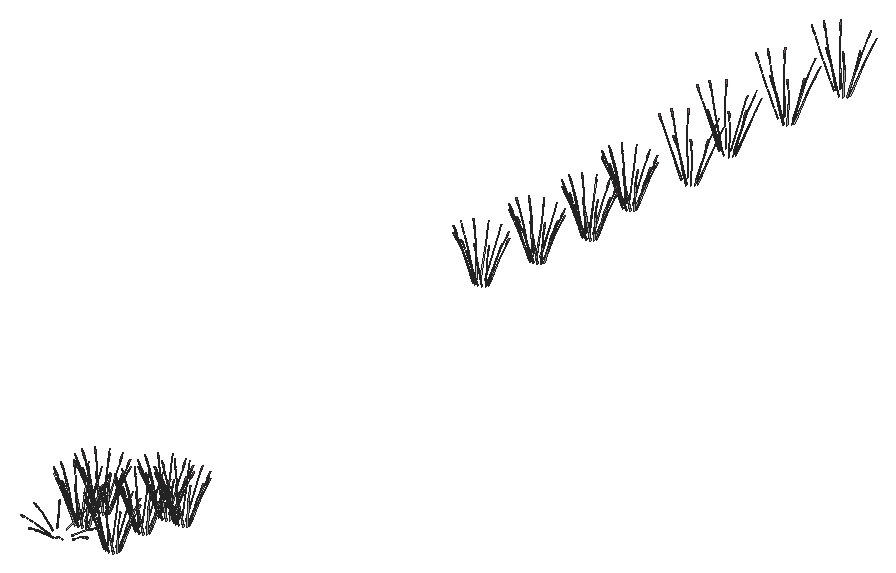
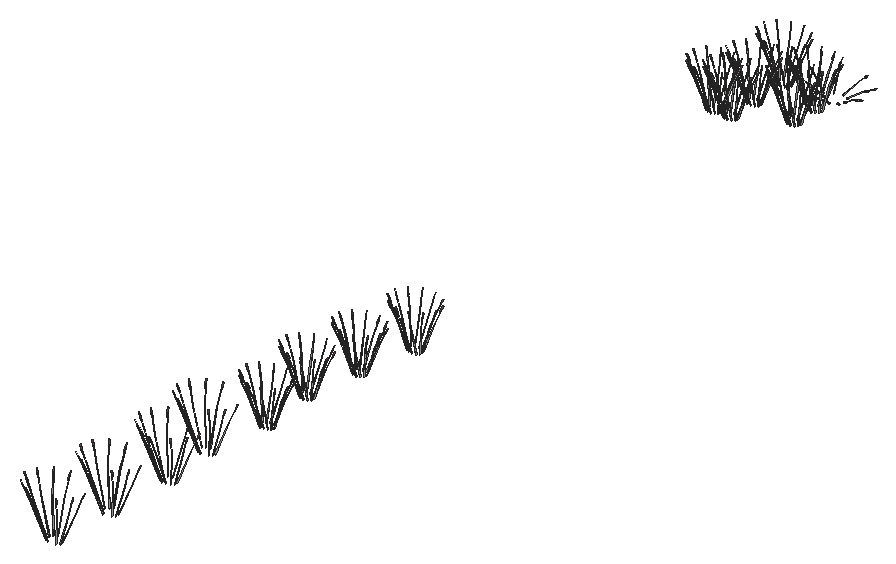
# SketchUp Ruby script. Lengths in inches.
U = 1.inch
M = Sketchup.active_model
def pt(a) = Geom::Point3d.new(a.map { |v| v * U })
def face(e, loops, mat)
  f = e.add_face(loops[0].map { |a| pt(a) })
  loops[1..].each { |l| e.add_face(l.map { |a| pt(a) }).erase! }
  f.material = f.back_material = mat if mat
  f
end
# faces: each face lists its corners as indices into pts; further lists are holes
def faces(e, pts, list, mat = nil) = list.each { |f| face(e, (f[0].is_a?(Array) ? f : [f]).map { |l| l.map { |i| pts[i] } }, mat) }
# xy, xz, yz: faces in a plane at the given z, y or x. An outline is a flat list of corners, or four numbers for a rectangle; further outlines are holes
def ring(l) = l.size == 4 ? [[l[0], l[1]], [l[2], l[1]], [l[2], l[3]], [l[0], l[3]]] : l.each_slice(2).to_a
def flat(e, list, mat, &to3) = list.each { |f| face(e, (f[0].is_a?(Array) ? f : [f]).map { |l| ring(l).map { |u, v| to3.(u, v) } }, mat) }
def xy(e, z, list, mat = nil) = flat(e, list, mat) { |x, y| [x, y, z] }
def xz(e, y, list, mat = nil) = flat(e, list, mat) { |x, z| [x, y, z] }
def yz(e, x, list, mat = nil) = flat(e, list, mat) { |y, z| [x, y, z] }
def lines(e, pts, list) = list.each { |a, b| e.add_line(pt(pts[a]), pt(pts[b])) }
# prism: a flat outline (further loops are holes) pulled along v
def prism(e, loops, v, mat = nil)
  f = face(e, loops, mat); d = Geom::Vector3d.new(v.map { |x| x * U })
  f.pushpull(f.normal.samedirection?(d) ? d.length : -d.length)
end
def box(e, o, s, mat = nil) = prism(e, [[o, [o[0] + s[0], o[1], o[2]], [o[0] + s[0], o[1] + s[1], o[2]], [o[0], o[1] + s[1], o[2]]]], [0, 0, s[2]], mat)
def at(x, y, z, deg = 0) = Geom::Transformation.translation(pt([x, y, z])) * Geom::Transformation.rotation(ORIGIN, Z_AXIS, deg.degrees)
def axes(o, x, y, z) = Geom::Transformation.new([*x, 0, *y, 0, *z, 0, *pt(o).to_a, 1])
def part(name) = M.definitions.add(name)
# library, detail: a bought-in or finely detailed component or shape, given as its bounding box
def library(name, o, s) = part(name).tap { |d| box(d.entities, o, s) }
def detail(e, o, s) = box(e.add_group.entities, o, s)
def put(e, d, t, mat = nil) = e.add_instance(d, t).tap { |i| i.material = mat if mat }
def group(e, t, mat = nil) = e.add_group.tap { |g| g.transformation = t; g.material = mat if mat }.entities
root = M.entities
M.materials.add("LightPink_Translucent").color = [144, 107, 117]
c1 = part("blade")
p = [[2.15,0.21,22],[0,0.17,0],[0.09,0.45,0],[2.18,0.31,22],[2.29,0.31,22],[0.38,0.45,0],
  [2.48,0.24,33],[2.49,0.24,33],[2.48,0.22,33]]
faces(c1.entities,p,[[0,1,2,3],[4,5,2,3],[6,3,4,7],[8,0,3,6]])
c2 = part("seeds")
p = [[0.3,-0.1,1.38],[-0.01,-0.03,1.59],[-0.01,-0.03,0.03],[0.14,-0.07,-0.07],[0.29,-0.03,3],[0.15,0.01,3.11]]
faces(c2.entities,p,[[0,1,2,3],[1,0,4,5]],"LightPink_Translucent")
c3 = part("blade with seeds")
put(c3.entities,c1,at(0,0,0))
put(c3.entities,c2,axes([2.4,0.25,30.99],[1.5799,-0.05474,1.17369],[-0.12525,1.92788,0.29478],[-0.07173,-0.02425,1.56792]))
put(root,c3,axes([53.96,597.61,46.73],[-0.90362,0.68241,0.48003],[-0.77932,-0.72471,0.3958],[0.42395,0.12588,0.9933]))
put(root,c3,axes([55.23,595.46,46.73],[-0.34623,0.9443,0.48003],[-1.13828,-0.3229,0.3958],[0.44763,-0.05675,0.9933]))
put(root,c3,axes([44.01,596.27,46.73],[-0.30393,-0.95317,0.48003],[1.19224,-0.16542,0.3958],[-0.35138,0.22417,0.9933]))
put(root,c3,axes([45.75,598.19,46.73],[-0.87265,-0.70663,0.48003],[0.92674,-0.60943,0.3958],[-0.16097,0.33153,0.9933]))
put(root,c3,axes([53.22,591.18,46.73],[0.87265,0.70663,0.48003],[-0.92674,0.60943,0.3958],[0.16097,-0.33153,0.9933]))
put(root,c3,axes([43.73,593.91,46.73],[0.34623,-0.9443,0.48003],[1.13828,0.3229,0.3958],[-0.44763,0.05675,0.9933]))
put(root,c3,axes([54.96,593.11,46.73],[0.30393,0.95317,0.48003],[-1.19224,0.16542,0.3958],[0.35138,-0.22417,0.9933]))
put(root,c3,axes([51.5,598.97,46.73],[-1.21888,0.23767,0.48003],[-0.21154,-0.93233,0.3958],[0.28666,0.27478,0.9933]))
put(root,c3,axes([53.27,639.2,46.73],[1.20755,0.27075,0.48003],[-0.41292,0.89013,0.3958],[-0.07257,-0.35005,0.9933]))
put(root,c3,axes([56.76,646.62,46.73],[-0.90362,0.68241,0.48003],[-0.77932,-0.72471,0.3958],[0.42395,0.12588,0.9933]))
put(root,c3,axes([58.02,644.47,46.73],[-0.34623,0.9443,0.48003],[-1.13828,-0.3229,0.3958],[0.44763,-0.05675,0.9933]))
put(root,c3,axes([46.8,645.27,46.73],[-0.30393,-0.95317,0.48003],[1.19224,-0.16542,0.3958],[-0.35138,0.22417,0.9933]))
put(root,c3,axes([48.54,647.2,46.73],[-0.87265,-0.70663,0.48003],[0.92674,-0.60943,0.3958],[-0.16097,0.33153,0.9933]))
put(root,c3,axes([56.01,640.19,46.73],[0.87265,0.70663,0.48003],[-0.92674,0.60943,0.3958],[0.16097,-0.33153,0.9933]))
put(root,c3,axes([46.52,642.92,46.73],[0.34623,-0.9443,0.48003],[1.13828,0.3229,0.3958],[-0.44763,0.05675,0.9933]))
put(root,c3,axes([57.75,642.12,46.73],[0.30393,0.95317,0.48003],[-1.19224,0.16542,0.3958],[0.35138,-0.22417,0.9933]))
put(root,c3,axes([54.29,647.98,46.73],[-1.21888,0.23767,0.48003],[-0.21154,-0.93233,0.3958],[0.28666,0.27478,0.9933]))
put(root,c3,axes([57.81,683.53,46.73],[1.20755,0.27075,0.48003],[-0.41292,0.89013,0.3958],[-0.07257,-0.35005,0.9933]))
put(root,c3,axes([61.3,690.95,46.73],[-0.90362,0.68241,0.48003],[-0.77932,-0.72471,0.3958],[0.42395,0.12588,0.9933]))
put(root,c3,axes([62.5625,688.8,46.73],[-0.34623,0.9443,0.48003],[-1.13828,-0.3229,0.3958],[0.44763,-0.05675,0.9933]))
put(root,c3,axes([51.34,689.6,46.73],[-0.30393,-0.95317,0.48003],[1.19224,-0.16542,0.3958],[-0.35138,0.22417,0.9933]))
put(root,c3,axes([53.08,691.53,46.73],[-0.87265,-0.70663,0.48003],[0.92674,-0.60943,0.3958],[-0.16097,0.33153,0.9933]))
put(root,c3,axes([60.55,684.52,46.73],[0.87265,0.70663,0.48003],[-0.92674,0.60943,0.3958],[0.16097,-0.33153,0.9933]))
put(root,c3,axes([51.06,687.25,46.73],[0.34623,-0.9443,0.48003],[1.13828,0.3229,0.3958],[-0.44763,0.05675,0.9933]))
put(root,c3,axes([62.29,686.45,46.73],[0.30393,0.95317,0.48003],[-1.19224,0.16542,0.3958],[0.35138,-0.22417,0.9933]))
put(root,c3,axes([58.83,692.31,46.73],[-1.21888,0.23767,0.48003],[-0.21154,-0.93233,0.3958],[0.28666,0.27478,0.9933]))
put(root,c3,axes([54.3,551.37,46.73],[1.20755,0.27075,0.48003],[-0.41292,0.89013,0.3958],[-0.07257,-0.35005,0.9933]))
put(root,c3,axes([57.79,558.78,46.73],[-0.90362,0.68241,0.48003],[-0.77932,-0.72471,0.3958],[0.42395,0.12588,0.9933]))
put(root,c3,axes([59.0625,556.64,46.73],[-0.34623,0.9443,0.48003],[-1.13828,-0.3229,0.3958],[0.44763,-0.05675,0.9933]))
put(root,c3,axes([47.84,557.44,46.73],[-0.30393,-0.95317,0.48003],[1.19224,-0.16542,0.3958],[-0.35138,0.22417,0.9933]))
put(root,c3,axes([49.58,559.37,46.73],[-0.87265,-0.70663,0.48003],[0.92674,-0.60943,0.3958],[-0.16097,0.33153,0.9933]))
put(root,c3,axes([57.05,552.36,46.73],[0.87265,0.70663,0.48003],[-0.92674,0.60943,0.3958],[0.16097,-0.33153,0.9933]))
put(root,c3,axes([47.5625,555.09,46.73],[0.34623,-0.9443,0.48003],[1.13828,0.3229,0.3958],[-0.44763,0.05675,0.9933]))
put(root,c3,axes([58.79,554.29,46.73],[0.30393,0.95317,0.48003],[-1.19224,0.16542,0.3958],[0.35138,-0.22417,0.9933]))
put(root,c3,axes([55.33,560.14,46.73],[-1.21888,0.23767,0.48003],[-0.21154,-0.93233,0.3958],[0.28666,0.27478,0.9933]))
put(root,c3,axes([23.85,22.0625,46.97],[-0.20012,0.13446,1.74944],[0.01702,0.98243,-0.27667],[-0.45871,0.12776,0.14031]))
put(root,c3,axes([39.17,21.75,46.97],[0.17006,-0.15775,1.74944],[-0.21766,-0.96766,-0.27667],[0.42669,-0.18347,0.14031]))
put(root,c3,axes([35.52,24.54,46.97],[0.26289,-0.01751,1.74944],[0.72108,-0.8046,-0.27667],[0.46761,0.10621,0.14031]))
put(root,c3,axes([35.54,17.54,46.97],[-0.01183,-0.20612,1.74944],[-0.99913,-0.59572,-0.27667],[0.15447,-0.36112,0.14031]))
put(root,c3,axes([23.89,25.73,46.97],[-0.03046,0.20495,1.74944],[0.86449,0.71297,-0.27667],[-0.22632,0.33716,0.14031]))
put(root,c3,axes([28.86,28.27,46.97],[0.15534,0.16677,1.74944],[1.25362,0.06552,-0.27667],[0.12606,0.3678,0.14031]))
put(root,c3,axes([29.92,15.76,46.97],[-0.18744,-0.14521,1.74944],[-1.25089,0.09206,-0.27667],[-0.19964,-0.34731,0.14031]))
put(root,c3,axes([25.82,17.35,46.97],[-0.26368,-0.00731,1.74944],[-0.83946,0.73103,-0.27667],[-0.44791,-0.14937,0.14031]))
put(root,c3,axes([31.05,42.08,47.05],[0.36946,-0.79643,0.35414],[1.07787,0.23229,-0.4572],[0.09883,0.32066,0.87481]))
put(root,c3,axes([33,34.39,47.05],[-0.36946,0.79643,0.35414],[-1.07787,-0.23229,-0.4572],[-0.09883,-0.32066,0.87481]))
put(root,c3,axes([35.79,40.82,47.05],[-0.69728,-0.64842,0.35414],[0.79619,-0.61382,-0.4572],[0.40453,0.09339,0.87481]))
put(root,c3,axes([36.94,39,47.05],[-1.01846,-0.28891,0.35414],[0.29705,-0.84289,-0.4572],[0.41005,-0.07729,0.87481]))
put(root,c3,axes([28.26,35.65,47.05],[0.69728,0.64842,0.35414],[-0.79619,0.61382,-0.4572],[-0.40453,-0.09339,0.87481]))
put(root,c3,axes([28.72,41.18,47.05],[0.82919,-0.54528,0.35414],[0.78493,0.62262,-0.4572],[-0.11943,0.31634,0.87481]))
put(root,c3,axes([27.28,39.49,47.05],[1.06674,-0.14801,0.35414],[0.28168,0.84611,-0.4572],[-0.30569,0.22726,0.87481]))
put(root,c3,axes([33.64,41.94,47.05],[-0.18927,-0.83419,0.35414],[1.08199,-0.22027,-0.4572],[0.29062,0.23905,0.87481]))
put(root,c3,axes([36.77,36.98,47.05],[-1.06674,0.14801,0.35414],[-0.28168,-0.84611,-0.4572],[0.30569,-0.22726,0.87481]))
put(root,c3,axes([27.11,37.47,47.05],[1.01846,0.28891,0.35414],[-0.29705,0.84289,-0.4572],[-0.41005,0.07729,0.87481]))
put(root,c3,axes([35.33,35.29,47.05],[-0.82919,0.54528,0.35414],[-0.78493,-0.62262,-0.4572],[0.11943,-0.31634,0.87481]))
put(root,c3,axes([30.42,34.53,47.05],[0.18927,0.83419,0.35414],[-1.08199,0.22027,-0.4572],[-0.29062,-0.23905,0.87481]))
put(root,c3,axes([30.75,61.11,47.05],[0.36946,-0.79643,0.35414],[1.07787,0.23229,-0.4572],[0.09883,0.32066,0.87481]))
put(root,c3,axes([32.71,53.42,47.05],[-0.36946,0.79643,0.35414],[-1.07787,-0.23229,-0.4572],[-0.09883,-0.32066,0.87481]))
put(root,c3,axes([35.49,59.85,47.05],[-0.69728,-0.64842,0.35414],[0.79619,-0.61382,-0.4572],[0.40453,0.09339,0.87481]))
put(root,c3,axes([36.64,58.03,47.05],[-1.01846,-0.28891,0.35414],[0.29705,-0.84289,-0.4572],[0.41005,-0.07729,0.87481]))
put(root,c3,axes([27.96,54.68,47.05],[0.69728,0.64842,0.35414],[-0.79619,0.61382,-0.4572],[-0.40453,-0.09339,0.87481]))
put(root,c3,axes([28.43,60.21,47.05],[0.82919,-0.54528,0.35414],[0.78493,0.62262,-0.4572],[-0.11943,0.31634,0.87481]))
put(root,c3,axes([26.99,58.52,47.05],[1.06674,-0.14801,0.35414],[0.28168,0.84611,-0.4572],[-0.30569,0.22726,0.87481]))
put(root,c3,axes([33.34,60.97,47.05],[-0.18927,-0.83419,0.35414],[1.08199,-0.22027,-0.4572],[0.29062,0.23905,0.87481]))
put(root,c3,axes([36.47,56.01,47.05],[-1.06674,0.14801,0.35414],[-0.28168,-0.84611,-0.4572],[0.30569,-0.22726,0.87481]))
put(root,c3,axes([26.82,56.5,47.05],[1.01846,0.28891,0.35414],[-0.29705,0.84289,-0.4572],[-0.41005,0.07729,0.87481]))
put(root,c3,axes([35.03,54.32,47.05],[-0.82919,0.54528,0.35414],[-0.78493,-0.62262,-0.4572],[0.11943,-0.31634,0.87481]))
put(root,c3,axes([30.12,53.55,47.05],[0.18927,0.83419,0.35414],[-1.08199,0.22027,-0.4572],[-0.29062,-0.23905,0.87481]))
put(root,c3,axes([62.52,30.08,47.05],[0.36946,-0.79643,0.35414],[1.07787,0.23229,-0.4572],[0.09883,0.32066,0.87481]))
put(root,c3,axes([64.48,22.39,47.05],[-0.36946,0.79643,0.35414],[-1.07787,-0.23229,-0.4572],[-0.09883,-0.32066,0.87481]))
put(root,c3,axes([67.26,28.82,47.05],[-0.69728,-0.64842,0.35414],[0.79619,-0.61382,-0.4572],[0.40453,0.09339,0.87481]))
put(root,c3,axes([68.41,27,47.05],[-1.01846,-0.28891,0.35414],[0.29705,-0.84289,-0.4572],[0.41005,-0.07729,0.87481]))
put(root,c3,axes([59.73,23.65,47.05],[0.69728,0.64842,0.35414],[-0.79619,0.61382,-0.4572],[-0.40453,-0.09339,0.87481]))
put(root,c3,axes([60.2,29.18,47.05],[0.82919,-0.54528,0.35414],[0.78493,0.62262,-0.4572],[-0.11943,0.31634,0.87481]))
put(root,c3,axes([58.76,27.49,47.05],[1.06674,-0.14801,0.35414],[0.28168,0.84611,-0.4572],[-0.30569,0.22726,0.87481]))
put(root,c3,axes([65.11,29.94,47.05],[-0.18927,-0.83419,0.35414],[1.08199,-0.22027,-0.4572],[0.29062,0.23905,0.87481]))
put(root,c3,axes([68.24,24.98,47.05],[-1.06674,0.14801,0.35414],[-0.28168,-0.84611,-0.4572],[0.30569,-0.22726,0.87481]))
put(root,c3,axes([58.59,25.47,47.05],[1.01846,0.28891,0.35414],[-0.29705,0.84289,-0.4572],[-0.41005,0.07729,0.87481]))
put(root,c3,axes([66.8,23.29,47.05],[-0.82919,0.54528,0.35414],[-0.78493,-0.62262,-0.4572],[0.11943,-0.31634,0.87481]))
put(root,c3,axes([61.89,22.53,47.05],[0.18927,0.83419,0.35414],[-1.08199,0.22027,-0.4572],[-0.29062,-0.23905,0.87481]))
put(root,c3,axes([62.3125,57.36,47.05],[0.36946,-0.79643,0.35414],[1.07787,0.23229,-0.4572],[0.09883,0.32066,0.87481]))
put(root,c3,axes([64.27,49.68,47.05],[-0.36946,0.79643,0.35414],[-1.07787,-0.23229,-0.4572],[-0.09883,-0.32066,0.87481]))
put(root,c3,axes([67.06,56.1,47.05],[-0.69728,-0.64842,0.35414],[0.79619,-0.61382,-0.4572],[0.40453,0.09339,0.87481]))
put(root,c3,axes([68.2,54.28,47.05],[-1.01846,-0.28891,0.35414],[0.29705,-0.84289,-0.4572],[0.41005,-0.07729,0.87481]))
put(root,c3,axes([59.53,50.9375,47.05],[0.69728,0.64842,0.35414],[-0.79619,0.61382,-0.4572],[-0.40453,-0.09339,0.87481]))
put(root,c3,axes([59.99,56.47,47.05],[0.82919,-0.54528,0.35414],[0.78493,0.62262,-0.4572],[-0.11943,0.31634,0.87481]))
put(root,c3,axes([58.55,54.78,47.05],[1.06674,-0.14801,0.35414],[0.28168,0.84611,-0.4572],[-0.30569,0.22726,0.87481]))
put(root,c3,axes([64.9,57.23,47.05],[-0.18927,-0.83419,0.35414],[1.08199,-0.22027,-0.4572],[0.29062,0.23905,0.87481]))
put(root,c3,axes([68.03,52.26,47.05],[-1.06674,0.14801,0.35414],[-0.28168,-0.84611,-0.4572],[0.30569,-0.22726,0.87481]))
put(root,c3,axes([58.38,52.76,47.05],[1.01846,0.28891,0.35414],[-0.29705,0.84289,-0.4572],[-0.41005,0.07729,0.87481]))
put(root,c3,axes([66.59,50.58,47.05],[-0.82919,0.54528,0.35414],[-0.78493,-0.62262,-0.4572],[0.11943,-0.31634,0.87481]))
put(root,c3,axes([61.68,49.8125,47.05],[0.18927,0.83419,0.35414],[-1.08199,0.22027,-0.4572],[-0.29062,-0.23905,0.87481]))
put(root,c3,axes([62.3125,78.08,47.05],[0.36946,-0.79643,0.35414],[1.07787,0.23229,-0.4572],[0.09883,0.32066,0.87481]))
put(root,c3,axes([64.27,70.39,47.05],[-0.36946,0.79643,0.35414],[-1.07787,-0.23229,-0.4572],[-0.09883,-0.32066,0.87481]))
put(root,c3,axes([67.06,76.82,47.05],[-0.69728,-0.64842,0.35414],[0.79619,-0.61382,-0.4572],[0.40453,0.09339,0.87481]))
put(root,c3,axes([68.2,75,47.05],[-1.01846,-0.28891,0.35414],[0.29705,-0.84289,-0.4572],[0.41005,-0.07729,0.87481]))
put(root,c3,axes([59.53,71.65,47.05],[0.69728,0.64842,0.35414],[-0.79619,0.61382,-0.4572],[-0.40453,-0.09339,0.87481]))
put(root,c3,axes([59.99,77.18,47.05],[0.82919,-0.54528,0.35414],[0.78493,0.62262,-0.4572],[-0.11943,0.31634,0.87481]))
put(root,c3,axes([58.55,75.49,47.05],[1.06674,-0.14801,0.35414],[0.28168,0.84611,-0.4572],[-0.30569,0.22726,0.87481]))
put(root,c3,axes([64.9,77.94,47.05],[-0.18927,-0.83419,0.35414],[1.08199,-0.22027,-0.4572],[0.29062,0.23905,0.87481]))
put(root,c3,axes([68.03,72.98,47.05],[-1.06674,0.14801,0.35414],[-0.28168,-0.84611,-0.4572],[0.30569,-0.22726,0.87481]))
put(root,c3,axes([58.38,73.47,47.05],[1.01846,0.28891,0.35414],[-0.29705,0.84289,-0.4572],[-0.41005,0.07729,0.87481]))
put(root,c3,axes([66.59,71.29,47.05],[-0.82919,0.54528,0.35414],[-0.78493,-0.62262,-0.4572],[0.11943,-0.31634,0.87481]))
put(root,c3,axes([61.68,70.53,47.05],[0.18927,0.83419,0.35414],[-1.08199,0.22027,-0.4572],[-0.29062,-0.23905,0.87481]))
put(root,c3,axes([74.3125,78.08,47.05],[0.36946,-0.79643,0.35414],[1.07787,0.23229,-0.4572],[0.09883,0.32066,0.87481]))
put(root,c3,axes([76.27,70.39,47.05],[-0.36946,0.79643,0.35414],[-1.07787,-0.23229,-0.4572],[-0.09883,-0.32066,0.87481]))
put(root,c3,axes([79.06,76.82,47.05],[-0.69728,-0.64842,0.35414],[0.79619,-0.61382,-0.4572],[0.40453,0.09339,0.87481]))
put(root,c3,axes([80.2,75,47.05],[-1.01846,-0.28891,0.35414],[0.29705,-0.84289,-0.4572],[0.41005,-0.07729,0.87481]))
put(root,c3,axes([71.53,71.65,47.05],[0.69728,0.64842,0.35414],[-0.79619,0.61382,-0.4572],[-0.40453,-0.09339,0.87481]))
put(root,c3,axes([71.99,77.18,47.05],[0.82919,-0.54528,0.35414],[0.78493,0.62262,-0.4572],[-0.11943,0.31634,0.87481]))
put(root,c3,axes([70.55,75.49,47.05],[1.06674,-0.14801,0.35414],[0.28168,0.84611,-0.4572],[-0.30569,0.22726,0.87481]))
put(root,c3,axes([76.9,77.94,47.05],[-0.18927,-0.83419,0.35414],[1.08199,-0.22027,-0.4572],[0.29062,0.23905,0.87481]))
put(root,c3,axes([80.03,72.98,47.05],[-1.06674,0.14801,0.35414],[-0.28168,-0.84611,-0.4572],[0.30569,-0.22726,0.87481]))
put(root,c3,axes([70.38,73.47,47.05],[1.01846,0.28891,0.35414],[-0.29705,0.84289,-0.4572],[-0.41005,0.07729,0.87481]))
put(root,c3,axes([78.59,71.29,47.05],[-0.82919,0.54528,0.35414],[-0.78493,-0.62262,-0.4572],[0.11943,-0.31634,0.87481]))
put(root,c3,axes([73.68,70.53,47.05],[0.18927,0.83419,0.35414],[-1.08199,0.22027,-0.4572],[-0.29062,-0.23905,0.87481]))
put(root,c3,axes([33.47,396.8125,47.05],[0.36946,-0.79643,0.35414],[1.07787,0.23229,-0.4572],[0.09883,0.32066,0.87481]))
put(root,c3,axes([35.43,389.13,47.05],[-0.36946,0.79643,0.35414],[-1.07787,-0.23229,-0.4572],[-0.09883,-0.32066,0.87481]))
put(root,c3,axes([38.22,395.56,47.05],[-0.69728,-0.64842,0.35414],[0.79619,-0.61382,-0.4572],[0.40453,0.09339,0.87481]))
put(root,c3,axes([39.36,393.74,47.05],[-1.01846,-0.28891,0.35414],[0.29705,-0.84289,-0.4572],[0.41005,-0.07729,0.87481]))
put(root,c3,axes([30.68,390.39,47.05],[0.69728,0.64842,0.35414],[-0.79619,0.61382,-0.4572],[-0.40453,-0.09339,0.87481]))
put(root,c3,axes([31.15,395.92,47.05],[0.82919,-0.54528,0.35414],[0.78493,0.62262,-0.4572],[-0.11943,0.31634,0.87481]))
put(root,c3,axes([29.71,394.23,47.05],[1.06674,-0.14801,0.35414],[0.28168,0.84611,-0.4572],[-0.30569,0.22726,0.87481]))
put(root,c3,axes([36.06,396.68,47.05],[-0.18927,-0.83419,0.35414],[1.08199,-0.22027,-0.4572],[0.29062,0.23905,0.87481]))
put(root,c3,axes([39.19,391.71,47.05],[-1.06674,0.14801,0.35414],[-0.28168,-0.84611,-0.4572],[0.30569,-0.22726,0.87481]))
put(root,c3,axes([29.54,392.21,47.05],[1.01846,0.28891,0.35414],[-0.29705,0.84289,-0.4572],[-0.41005,0.07729,0.87481]))
put(root,c3,axes([37.75,390.03,47.05],[-0.82919,0.54528,0.35414],[-0.78493,-0.62262,-0.4572],[0.11943,-0.31634,0.87481]))
put(root,c3,axes([32.84,389.26,47.05],[0.18927,0.83419,0.35414],[-1.08199,0.22027,-0.4572],[-0.29062,-0.23905,0.87481]))
put(root,c3,axes([41.625,436.51,47.05],[0.36946,-0.79643,0.35414],[1.07787,0.23229,-0.4572],[0.09883,0.32066,0.87481]))
put(root,c3,axes([43.58,428.82,47.05],[-0.36946,0.79643,0.35414],[-1.07787,-0.23229,-0.4572],[-0.09883,-0.32066,0.87481]))
put(root,c3,axes([46.37,435.25,47.05],[-0.69728,-0.64842,0.35414],[0.79619,-0.61382,-0.4572],[0.40453,0.09339,0.87481]))
put(root,c3,axes([47.52,433.43,47.05],[-1.01846,-0.28891,0.35414],[0.29705,-0.84289,-0.4572],[0.41005,-0.07729,0.87481]))
put(root,c3,axes([38.84,430.08,47.05],[0.69728,0.64842,0.35414],[-0.79619,0.61382,-0.4572],[-0.40453,-0.09339,0.87481]))
put(root,c3,axes([39.3,435.61,47.05],[0.82919,-0.54528,0.35414],[0.78493,0.62262,-0.4572],[-0.11943,0.31634,0.87481]))
put(root,c3,axes([37.86,433.92,47.05],[1.06674,-0.14801,0.35414],[0.28168,0.84611,-0.4572],[-0.30569,0.22726,0.87481]))
put(root,c3,axes([44.21,436.375,47.05],[-0.18927,-0.83419,0.35414],[1.08199,-0.22027,-0.4572],[0.29062,0.23905,0.87481]))
put(root,c3,axes([47.35,431.41,47.05],[-1.06674,0.14801,0.35414],[-0.28168,-0.84611,-0.4572],[0.30569,-0.22726,0.87481]))
put(root,c3,axes([37.69,431.9,47.05],[1.01846,0.28891,0.35414],[-0.29705,0.84289,-0.4572],[-0.41005,0.07729,0.87481]))
put(root,c3,axes([45.91,429.72,47.05],[-0.82919,0.54528,0.35414],[-0.78493,-0.62262,-0.4572],[0.11943,-0.31634,0.87481]))
put(root,c3,axes([40.99,428.96,47.05],[0.18927,0.83419,0.35414],[-1.08199,0.22027,-0.4572],[-0.29062,-0.23905,0.87481]))
put(root,c3,axes([47.98,475.77,47.05],[0.36946,-0.79643,0.35414],[1.07787,0.23229,-0.4572],[0.09883,0.32066,0.87481]))
put(root,c3,axes([49.9375,468.09,47.05],[-0.36946,0.79643,0.35414],[-1.07787,-0.23229,-0.4572],[-0.09883,-0.32066,0.87481]))
put(root,c3,axes([52.72,474.51,47.05],[-0.69728,-0.64842,0.35414],[0.79619,-0.61382,-0.4572],[0.40453,0.09339,0.87481]))
put(root,c3,axes([53.87,472.69,47.05],[-1.01846,-0.28891,0.35414],[0.29705,-0.84289,-0.4572],[0.41005,-0.07729,0.87481]))
put(root,c3,axes([45.19,469.35,47.05],[0.69728,0.64842,0.35414],[-0.79619,0.61382,-0.4572],[-0.40453,-0.09339,0.87481]))
put(root,c3,axes([45.66,474.875,47.05],[0.82919,-0.54528,0.35414],[0.78493,0.62262,-0.4572],[-0.11943,0.31634,0.87481]))
put(root,c3,axes([44.22,473.1875,47.05],[1.06674,-0.14801,0.35414],[0.28168,0.84611,-0.4572],[-0.30569,0.22726,0.87481]))
put(root,c3,axes([50.57,475.64,47.05],[-0.18927,-0.83419,0.35414],[1.08199,-0.22027,-0.4572],[0.29062,0.23905,0.87481]))
put(root,c3,axes([53.7,470.67,47.05],[-1.06674,0.14801,0.35414],[-0.28168,-0.84611,-0.4572],[0.30569,-0.22726,0.87481]))
put(root,c3,axes([44.05,471.17,47.05],[1.01846,0.28891,0.35414],[-0.29705,0.84289,-0.4572],[-0.41005,0.07729,0.87481]))
put(root,c3,axes([52.26,468.99,47.05],[-0.82919,0.54528,0.35414],[-0.78493,-0.62262,-0.4572],[0.11943,-0.31634,0.87481]))
put(root,c3,axes([47.35,468.22,47.05],[0.18927,0.83419,0.35414],[-1.08199,0.22027,-0.4572],[-0.29062,-0.23905,0.87481]))
put(root,c3,axes([44.37,516.03,47.05],[0.36946,-0.79643,0.35414],[1.07787,0.23229,-0.4572],[0.09883,0.32066,0.87481]))
put(root,c3,axes([46.32,508.35,47.05],[-0.36946,0.79643,0.35414],[-1.07787,-0.23229,-0.4572],[-0.09883,-0.32066,0.87481]))
put(root,c3,axes([49.11,514.77,47.05],[-0.69728,-0.64842,0.35414],[0.79619,-0.61382,-0.4572],[0.40453,0.09339,0.87481]))
put(root,c3,axes([50.26,512.95,47.05],[-1.01846,-0.28891,0.35414],[0.29705,-0.84289,-0.4572],[0.41005,-0.07729,0.87481]))
put(root,c3,axes([41.58,509.61,47.05],[0.69728,0.64842,0.35414],[-0.79619,0.61382,-0.4572],[-0.40453,-0.09339,0.87481]))
put(root,c3,axes([42.04,515.13,47.05],[0.82919,-0.54528,0.35414],[0.78493,0.62262,-0.4572],[-0.11943,0.31634,0.87481]))
put(root,c3,axes([40.6,513.45,47.05],[1.06674,-0.14801,0.35414],[0.28168,0.84611,-0.4572],[-0.30569,0.22726,0.87481]))
put(root,c3,axes([46.95,515.9,47.05],[-0.18927,-0.83419,0.35414],[1.08199,-0.22027,-0.4572],[0.29062,0.23905,0.87481]))
put(root,c3,axes([50.09,510.93,47.05],[-1.06674,0.14801,0.35414],[-0.28168,-0.84611,-0.4572],[0.30569,-0.22726,0.87481]))
put(root,c3,axes([40.43,511.42,47.05],[1.01846,0.28891,0.35414],[-0.29705,0.84289,-0.4572],[-0.41005,0.07729,0.87481]))
put(root,c3,axes([48.65,509.24,47.05],[-0.82919,0.54528,0.35414],[-0.78493,-0.62262,-0.4572],[0.11943,-0.31634,0.87481]))
put(root,c3,axes([43.73,508.48,47.05],[0.18927,0.83419,0.35414],[-1.08199,0.22027,-0.4572],[-0.29062,-0.23905,0.87481]))
put(root,c3,axes([48.5,598.53,47.05],[0.36946,-0.79643,0.35414],[1.07787,0.23229,-0.4572],[0.09883,0.32066,0.87481]))
put(root,c3,axes([50.46,590.85,47.05],[-0.36946,0.79643,0.35414],[-1.07787,-0.23229,-0.4572],[-0.09883,-0.32066,0.87481]))
